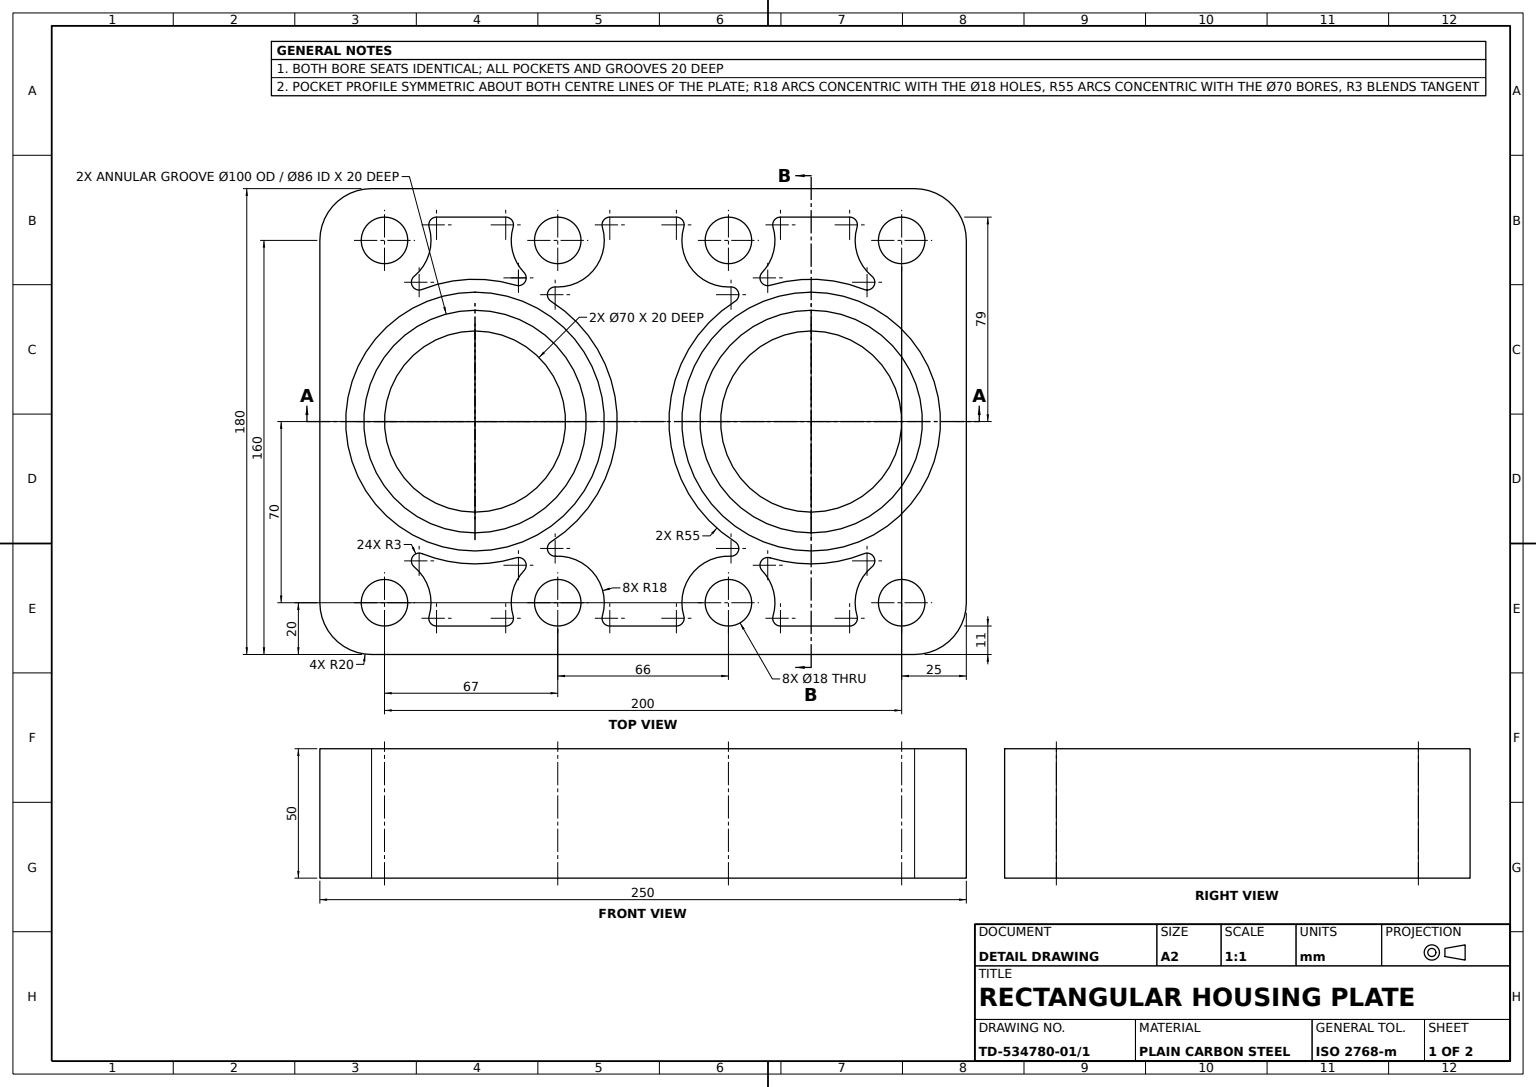
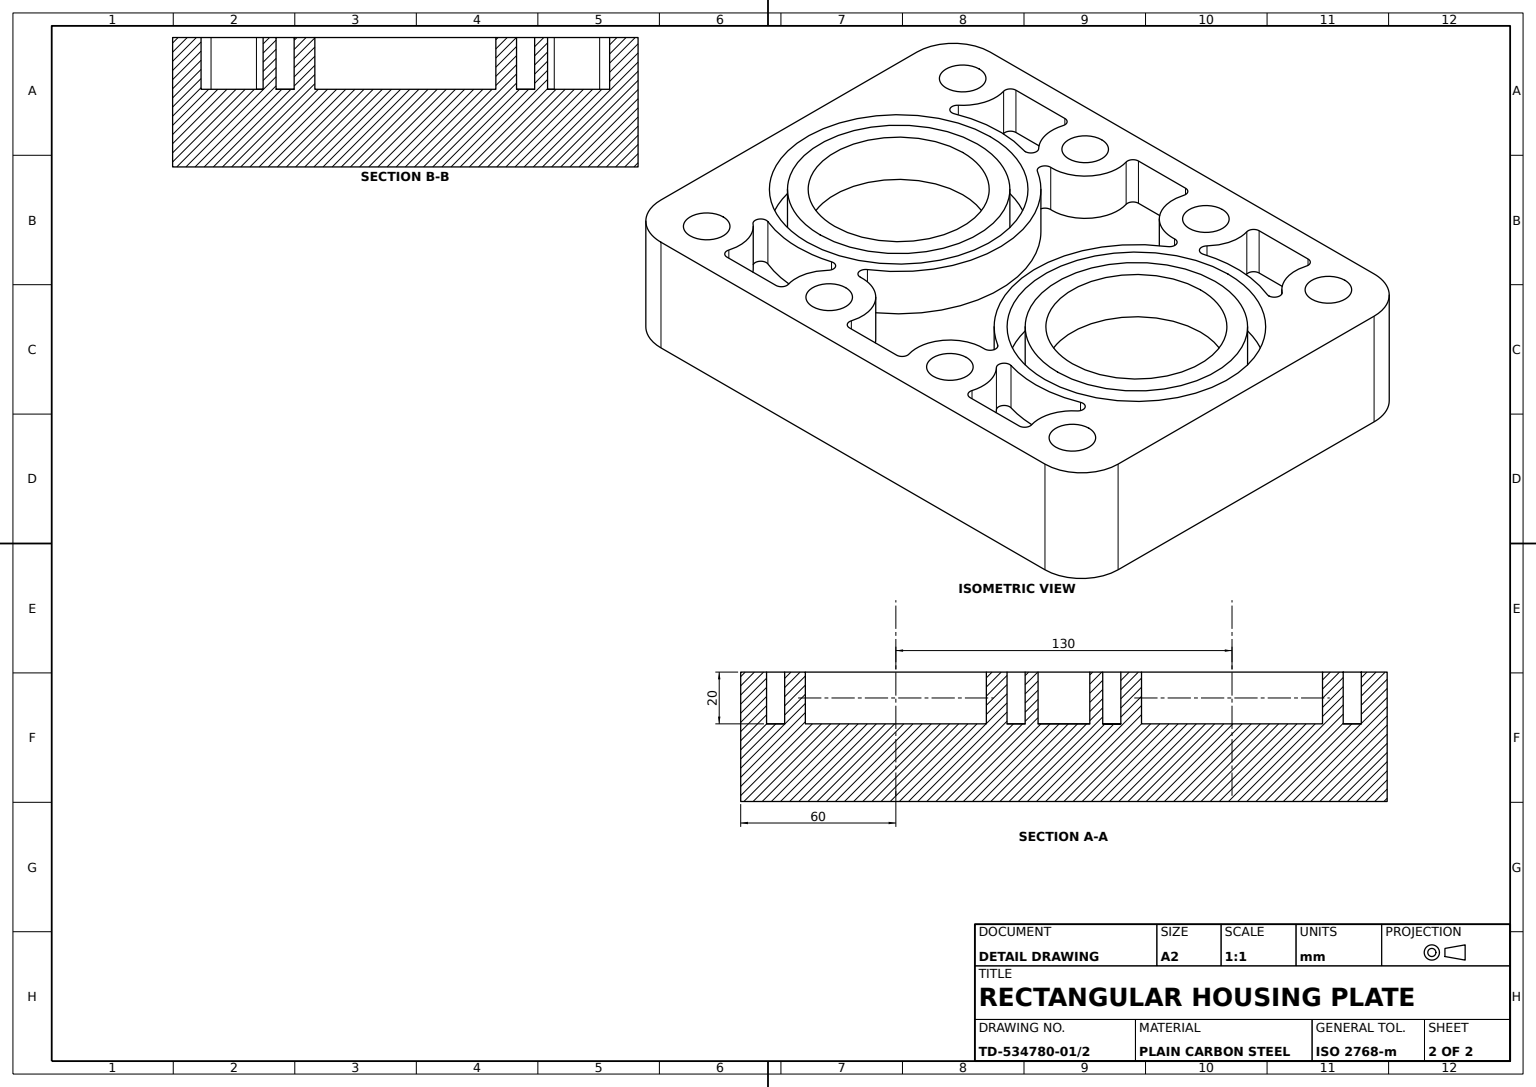
solid
v1 (100,0,61)
v2 (100,50,61)
e1 v1 v2 LINE
v3 (100,50,79)
e2 v2 v3 CIRCLE(AX(P(100,50,70),D(0,1,0),D(0,0,1)),9)
v4 (100,0,79)
e3 v4 v3 LINE
e4 v1 v4 CIRCLE(AX(P(100,0,70),D(0,1,0),D(0,0,1)),9)
face CYL(AX(P(100,-150,70),D(0,1,0),D(0,0,1)),9) rev [e1 e2 -e3 -e4]
v5 (65,30,-35)
v6 (65,30,35)
e5 v5 v6 CIRCLE(AX(P(65,30,0),D(0,1,0),D(0,0,1)),35)
e6 v6 v5 CIRCLE(AX(P(65,30,0),D(0,1,0),D(0,0,1)),35)
face PLANE(AX(P(0,30,0),D(0,1,0),D(0,0,1))) [e5 e6]
v7 (48.204819,30,-52.51506)
v8 (48.204819,50,-52.51506)
e7 v7 v8 LINE
v9 (49.073535,50,-52.643591)
e8 v8 v9 CIRCLE(AX(P(48.204819,50,-55.51506),D(0,1,0),D(0,0,1)),3)
v10 (49.073535,30,-52.643591)
e9 v10 v9 LINE
e10 v7 v10 CIRCLE(AX(P(48.204819,30,-55.51506),D(0,1,0),D(0,0,1)),3)
face CYL(AX(P(48.204819,30,-55.51506),D(0,1,0),D(0,0,1)),3) rev [e7 e8 -e9 -e10]
v11 (-125,50,-70)
v12 (-125,0,-70)
e11 v11 v12 LINE
v13 (-125,0,70)
e12 v12 v13 LINE
v14 (-125,50,70)
e13 v13 v14 LINE
e14 v11 v14 LINE
face PLANE(AX(P(-125,50,-90),D(1,0,0),D(0,0,-1))) rev [e11 e12 e13 -e14]
v15 (-33,0,61)
v16 (-33,50,61)
e15 v15 v16 LINE
v17 (-33,50,79)
e16 v16 v17 CIRCLE(AX(P(-33,50,70),D(0,1,0),D(0,0,1)),9)
v18 (-33,0,79)
e17 v18 v17 LINE
e18 v15 v18 CIRCLE(AX(P(-33,0,70),D(0,1,0),D(0,0,1)),9)
face CYL(AX(P(-33,-150,70),D(0,1,0),D(0,0,1)),9) rev [e15 e16 -e17 -e18]
v19 (-65,50,-35)
v20 (-65,50,35)
e19 v19 v20 CIRCLE(AX(P(-65,50,0),D(0,1,0),D(0,0,1)),35)
v21 (-65,30,35)
e20 v21 v20 LINE
v22 (-65,30,-35)
e21 v22 v21 CIRCLE(AX(P(-65,30,0),D(0,1,0),D(0,0,1)),35)
e22 v22 v19 LINE
face CYL(AX(P(-65,30,0),D(0,1,0),D(0,0,1)),35) rev [e19 -e20 -e21 e22]
v23 (-100,0,-61)
v24 (-100,50,-61)
e23 v23 v24 LINE
v25 (-100,50,-79)
e24 v24 v25 CIRCLE(AX(P(-100,50,-70),D(0,1,0),D(0,0,1)),9)
v26 (-100,0,-79)
e25 v26 v25 LINE
e26 v23 v26 CIRCLE(AX(P(-100,0,-70),D(0,1,0),D(0,0,1)),9)
face CYL(AX(P(-100,-150,-70),D(0,1,0),D(0,0,1)),9) rev [e23 e24 -e25 -e26]
v27 (-46.032702,30,57.584337)
v28 (-46.032702,50,57.584337)
e27 v27 v28 LINE
v29 (-49.073535,50,52.643591)
e28 v29 v28 CIRCLE(AX(P(-48.204819,50,55.51506),D(0,-1,0),D(0,0,1)),3)
v30 (-49.073535,30,52.643591)
e29 v30 v29 LINE
e30 v30 v27 CIRCLE(AX(P(-48.204819,30,55.51506),D(0,-1,0),D(0,0,1)),3)
face CYL(AX(P(-48.204819,30,55.51506),D(0,1,0),D(0,0,1)),3) rev [e27 -e28 -e29 e30]
v31 (-79.875388,30,79)
v32 (-79.875388,50,79)
e31 v31 v32 LINE
v33 (-82.750333,30,75.142857)
e32 v31 v33 CIRCLE(AX(P(-79.875388,30,76),D(0,-1,0),D(0,0,1)),3)
v34 (-82.750333,50,75.142857)
e33 v33 v34 LINE
e34 v32 v34 CIRCLE(AX(P(-79.875388,50,76),D(0,-1,0),D(0,0,1)),3)
face CYL(AX(P(-79.875388,30,76),D(0,1,0),D(0,0,1)),3) rev [-e31 e32 e33 -e34]
v35 (65,30,43)
v36 (65,30,-43)
e35 v35 v36 CIRCLE(AX(P(65,30,0),D(0,1,0),D(0,0,1)),43)
e36 v36 v35 CIRCLE(AX(P(65,30,0),D(0,1,0),D(0,0,1)),43)
v37 (65,30,50)
v38 (65,30,-50)
e37 v37 v38 CIRCLE(AX(P(65,30,0),D(0,1,0),D(0,0,1)),50)
e38 v38 v37 CIRCLE(AX(P(65,30,0),D(0,1,0),D(0,0,1)),50)
face PLANE(AX(P(0,30,0),D(0,1,0),D(0,0,1))) [-e35 -e36] [e37 e38]
v39 (35.608995,30,-46.488373)
v40 (35.608995,30,46.488373)
e39 v39 v40 CIRCLE(AX(P(65,30,0),D(0,1,0),D(0,0,1)),55)
v41 (35.608995,50,46.488373)
e40 v40 v41 LINE
v42 (35.608995,50,-46.488373)
e41 v42 v41 CIRCLE(AX(P(65,50,0),D(0,1,0),D(0,0,1)),55)
e42 v39 v42 LINE
face CYL(AX(P(65,30,0),D(0,1,0),D(0,0,1)),55) [e39 e40 -e41 -e42]
v43 (-48.204819,30,-52.51506)
v44 (-48.204819,50,-52.51506)
e43 v43 v44 LINE
v45 (-49.073535,30,-52.643591)
e44 v45 v43 CIRCLE(AX(P(-48.204819,30,-55.51506),D(0,1,0),D(0,0,1)),3)
v46 (-49.073535,50,-52.643591)
e45 v45 v46 LINE
e46 v46 v44 CIRCLE(AX(P(-48.204819,50,-55.51506),D(0,1,0),D(0,0,1)),3)
face CYL(AX(P(-48.204819,30,-55.51506),D(0,1,0),D(0,0,1)),3) rev [-e43 -e44 e45 e46]
v47 (33,0,-79)
v48 (33,50,-79)
e47 v47 v48 LINE
v49 (33,0,-61)
e48 v49 v47 CIRCLE(AX(P(33,0,-70),D(0,1,0),D(0,0,1)),9)
v50 (33,50,-61)
e49 v49 v50 LINE
e50 v50 v48 CIRCLE(AX(P(33,50,-70),D(0,1,0),D(0,0,1)),9)
face CYL(AX(P(33,-150,-70),D(0,1,0),D(0,0,1)),9) rev [-e47 -e48 e49 e50]
v51 (-50.249667,30,75.142857)
v52 (-53.124612,30,79)
e51 v51 v52 CIRCLE(AX(P(-53.124612,30,76),D(0,-1,0),D(0,0,1)),3)
e52 v27 v51 CIRCLE(AX(P(-33,30,70),D(0,1,0),D(0,0,1)),18)
v53 (-65,30,55)
e53 v53 v30 CIRCLE(AX(P(-65,30,0),D(0,1,0),D(0,0,1)),55)
v54 (-85.489465,30,51.040982)
e54 v54 v53 CIRCLE(AX(P(-65,30,0),D(0,1,0),D(0,0,1)),55)
v55 (-88.520347,30,56.135745)
e55 v55 v54 CIRCLE(AX(P(-86.607072,30,53.825035),D(0,-1,0),D(0,0,1)),3)
e56 v33 v55 CIRCLE(AX(P(-100,30,70),D(0,1,0),D(0,0,1)),18)
e57 v52 v31 LINE
face PLANE(AX(P(0,30,0),D(0,1,0),D(0,0,1))) [-e51 -e52 -e30 -e53 -e54 -e55 -e56 -e32 -e57]
v56 (65,30,55)
v57 (85.489465,30,51.040982)
e58 v56 v57 CIRCLE(AX(P(65,30,0),D(0,1,0),D(0,0,1)),55)
v58 (85.489465,50,51.040982)
e59 v57 v58 LINE
v59 (65,50,55)
e60 v59 v58 CIRCLE(AX(P(65,50,0),D(0,1,0),D(0,0,1)),55)
e61 v56 v59 LINE
face CYL(AX(P(65,30,0),D(0,1,0),D(0,0,1)),55) [e58 e59 -e60 -e61]
v60 (88.520347,30,56.135745)
e62 v57 v60 CIRCLE(AX(P(86.607072,30,53.825035),D(0,-1,0),D(0,0,1)),3)
v61 (88.520347,50,56.135745)
e63 v60 v61 LINE
e64 v58 v61 CIRCLE(AX(P(86.607072,50,53.825035),D(0,-1,0),D(0,0,1)),3)
face CYL(AX(P(86.607072,30,53.825035),D(0,1,0),D(0,0,1)),3) rev [-e59 e62 e63 -e64]
v62 (-35.608995,30,-46.488373)
v63 (-35.608995,50,-46.488373)
e65 v62 v63 LINE
v64 (-35.608995,50,46.488373)
e66 v64 v63 CIRCLE(AX(P(-65,50,0),D(0,1,0),D(0,0,1)),55)
v65 (-35.608995,30,46.488373)
e67 v65 v64 LINE
e68 v65 v62 CIRCLE(AX(P(-65,30,0),D(0,1,0),D(0,0,1)),55)
face CYL(AX(P(-65,30,0),D(0,1,0),D(0,0,1)),55) [e65 -e66 -e67 e68]
v66 (65,50,43)
e69 v35 v66 LINE
v67 (65,50,-43)
e70 v67 v66 CIRCLE(AX(P(65,50,0),D(0,1,0),D(0,0,1)),43)
e71 v36 v67 LINE
face CYL(AX(P(65,30,0),D(0,1,0),D(0,0,1)),43) [e36 e69 -e70 -e71]
v68 (15.750333,30,-75.142857)
v69 (12.875388,30,-79)
e72 v68 v69 CIRCLE(AX(P(12.875388,30,-76),D(0,1,0),D(0,0,1)),3)
v70 (15.750333,50,-75.142857)
e73 v68 v70 LINE
v71 (12.875388,50,-79)
e74 v70 v71 CIRCLE(AX(P(12.875388,50,-76),D(0,1,0),D(0,0,1)),3)
e75 v69 v71 LINE
face CYL(AX(P(12.875388,30,-76),D(0,1,0),D(0,0,1)),3) rev [-e72 e73 e74 -e75]
v72 (33,0,79)
v73 (33,50,79)
e76 v72 v73 LINE
v74 (33,50,61)
e77 v73 v74 CIRCLE(AX(P(33,50,70),D(0,1,0),D(0,0,1)),9)
v75 (33,0,61)
e78 v75 v74 LINE
e79 v72 v75 CIRCLE(AX(P(33,0,70),D(0,1,0),D(0,0,1)),9)
face CYL(AX(P(33,-150,70),D(0,1,0),D(0,0,1)),9) rev [e76 e77 -e78 -e79]
v76 (53.124612,30,-79)
v77 (50.249667,30,-75.142857)
e80 v76 v77 CIRCLE(AX(P(53.124612,30,-76),D(0,1,0),D(0,0,1)),3)
v78 (46.032702,30,-57.584337)
e81 v78 v77 CIRCLE(AX(P(33,30,-70),D(0,1,0),D(0,0,1)),18)
e82 v78 v7 CIRCLE(AX(P(48.204819,30,-55.51506),D(0,1,0),D(0,0,1)),3)
v79 (85.489465,30,-51.040982)
e83 v79 v10 CIRCLE(AX(P(65,30,0),D(0,1,0),D(0,0,1)),55)
v80 (86.607072,30,-50.825035)
e84 v79 v80 CIRCLE(AX(P(86.607072,30,-53.825035),D(0,1,0),D(0,0,1)),3)
v81 (88.520347,30,-56.135745)
e85 v80 v81 CIRCLE(AX(P(86.607072,30,-53.825035),D(0,1,0),D(0,0,1)),3)
v82 (82.750333,30,-75.142857)
e86 v82 v81 CIRCLE(AX(P(100,30,-70),D(0,1,0),D(0,0,1)),18)
v83 (79.875388,30,-79)
e87 v82 v83 CIRCLE(AX(P(79.875388,30,-76),D(0,1,0),D(0,0,1)),3)
e88 v76 v83 LINE
face PLANE(AX(P(0,30,0),D(0,1,0),D(0,0,1))) [e80 -e81 e82 e10 -e83 e84 e85 -e86 e87 -e88]
v84 (65,50,50)
v85 (65,50,-50)
e89 v84 v85 CIRCLE(AX(P(65,50,0),D(0,1,0),D(0,0,1)),50)
e90 v38 v85 LINE
e91 v37 v84 LINE
face CYL(AX(P(65,30,0),D(0,1,0),D(0,0,1)),50) rev [e89 -e90 -e37 e91]
v86 (-65,30,-50)
v87 (-65,30,50)
e92 v86 v87 CIRCLE(AX(P(-65,30,0),D(0,1,0),D(0,0,1)),50)
e93 v87 v86 CIRCLE(AX(P(-65,30,0),D(0,1,0),D(0,0,1)),50)
v88 (-65,30,-43)
v89 (-65,30,43)
e94 v88 v89 CIRCLE(AX(P(-65,30,0),D(0,1,0),D(0,0,1)),43)
e95 v89 v88 CIRCLE(AX(P(-65,30,0),D(0,1,0),D(0,0,1)),43)
face PLANE(AX(P(0,30,0),D(0,1,0),D(0,0,1))) [e92 e93] [-e94 -e95]
v90 (-33,50,-52)
v91 (-33.862157,50,-52.020659)
e96 v90 v91 CIRCLE(AX(P(-33,50,-70),D(0,-1,0),D(0,0,1)),18)
v92 (-33.862157,30,-52.020659)
e97 v92 v91 LINE
v93 (-33,30,-52)
e98 v93 v92 CIRCLE(AX(P(-33,30,-70),D(0,-1,0),D(0,0,1)),18)
e99 v93 v90 LINE
face CYL(AX(P(-33,30,-70),D(0,1,0),D(0,0,1)),18) [e96 -e97 -e98 e99]
v94 (-53.124612,50,79)
e100 v94 v32 LINE
e101 v52 v94 LINE
face PLANE(AX(P(0,30,79),D(0,0,-1),D(-1,0,0))) [e57 e31 -e100 -e101]
v95 (65,50,-35)
e102 v5 v95 LINE
v96 (65,50,35)
e103 v6 v96 LINE
e104 v96 v95 CIRCLE(AX(P(65,50,0),D(0,1,0),D(0,0,1)),35)
face CYL(AX(P(65,30,0),D(0,1,0),D(0,0,1)),35) rev [-e102 -e6 e103 e104]
v97 (-50.249667,50,75.142857)
e105 v97 v94 CIRCLE(AX(P(-53.124612,50,76),D(0,-1,0),D(0,0,1)),3)
e106 v51 v97 LINE
face CYL(AX(P(-53.124612,30,76),D(0,1,0),D(0,0,1)),3) rev [-e105 -e106 e51 e101]
v98 (88.520347,50,-56.135745)
e107 v81 v98 LINE
v99 (86.607072,50,-50.825035)
e108 v80 v99 LINE
e109 v99 v98 CIRCLE(AX(P(86.607072,50,-53.825035),D(0,1,0),D(0,0,1)),3)
face CYL(AX(P(86.607072,30,-53.825035),D(0,1,0),D(0,0,1)),3) rev [-e107 -e85 e108 e109]
e110 v21 v22 CIRCLE(AX(P(-65,30,0),D(0,1,0),D(0,0,1)),35)
e111 v20 v19 CIRCLE(AX(P(-65,50,0),D(0,1,0),D(0,0,1)),35)
face CYL(AX(P(-65,30,0),D(0,1,0),D(0,0,1)),35) rev [-e110 e20 e111 -e22]
e112 v47 v49 CIRCLE(AX(P(33,0,-70),D(0,1,0),D(0,0,1)),9)
e113 v48 v50 CIRCLE(AX(P(33,50,-70),D(0,1,0),D(0,0,1)),9)
face CYL(AX(P(33,-150,-70),D(0,1,0),D(0,0,1)),9) rev [-e49 -e112 e47 e113]
v100 (-12.875388,50,-79)
e114 v100 v71 LINE
v101 (-12.875388,30,-79)
e115 v101 v100 LINE
e116 v101 v69 LINE
face PLANE(AX(P(0,30,-79),D(0,0,1),D(1,0,0))) [e75 -e114 -e115 e116]
v102 (33.862157,50,-52.020659)
e117 v42 v102 CIRCLE(AX(P(34.00585,50,-49.024103),D(0,1,0),D(0,0,1)),3)
v103 (33.862157,30,-52.020659)
e118 v103 v102 LINE
e119 v39 v103 CIRCLE(AX(P(34.00585,30,-49.024103),D(0,1,0),D(0,0,1)),3)
face CYL(AX(P(34.00585,30,-49.024103),D(0,1,0),D(0,0,1)),3) rev [e42 e117 -e118 -e119]
v104 (-65,50,55)
e120 v104 v29 CIRCLE(AX(P(-65,50,0),D(0,1,0),D(0,0,1)),55)
e121 v53 v104 LINE
face CYL(AX(P(-65,30,0),D(0,1,0),D(0,0,1)),55) [e29 -e120 -e121 e53]
v105 (-34.00585,30,52.024103)
e122 v105 v65 CIRCLE(AX(P(-34.00585,30,49.024103),D(0,-1,0),D(0,0,1)),3)
v106 (-34.00585,50,52.024103)
e123 v106 v64 CIRCLE(AX(P(-34.00585,50,49.024103),D(0,-1,0),D(0,0,1)),3)
e124 v105 v106 LINE
face CYL(AX(P(-34.00585,30,49.024103),D(0,1,0),D(0,0,1)),3) rev [e122 e67 -e123 -e124]
v107 (105,50,-90)
v108 (105,0,-90)
e125 v107 v108 LINE
v109 (-105,0,-90)
e126 v108 v109 LINE
v110 (-105,50,-90)
e127 v109 v110 LINE
e128 v107 v110 LINE
face PLANE(AX(P(125,50,-90),D(0,0,1),D(1,0,0))) rev [e125 e126 e127 -e128]
v111 (-100,0,79)
v112 (-100,50,79)
e129 v111 v112 LINE
v113 (-100,50,61)
e130 v112 v113 CIRCLE(AX(P(-100,50,70),D(0,1,0),D(0,0,1)),9)
v114 (-100,0,61)
e131 v114 v113 LINE
e132 v111 v114 CIRCLE(AX(P(-100,0,70),D(0,1,0),D(0,0,1)),9)
face CYL(AX(P(-100,-150,70),D(0,1,0),D(0,0,1)),9) rev [e129 e130 -e131 -e132]
v115 (-79.875388,30,-79)
v116 (-79.875388,50,-79)
e133 v115 v116 LINE
v117 (-53.124612,30,-79)
e134 v117 v115 LINE
v118 (-53.124612,50,-79)
e135 v117 v118 LINE
e136 v118 v116 LINE
face PLANE(AX(P(0,30,-79),D(0,0,-1),D(-1,0,0))) rev [-e133 -e134 e135 e136]
v119 (85.489465,50,-51.040982)
e137 v119 v9 CIRCLE(AX(P(65,50,0),D(0,1,0),D(0,0,1)),55)
e138 v79 v119 LINE
face CYL(AX(P(65,30,0),D(0,1,0),D(0,0,1)),55) [e83 e9 -e137 -e138]
e139 v66 v67 CIRCLE(AX(P(65,50,0),D(0,1,0),D(0,0,1)),43)
e140 v95 v96 CIRCLE(AX(P(65,50,0),D(0,1,0),D(0,0,1)),35)
face PLANE(AX(P(0,50,0),D(0,1,0),D(0,0,1))) [e70 e139] [-e104 -e140]
v120 (53.124612,30,79)
v121 (53.124612,50,79)
e141 v120 v121 LINE
v122 (50.249667,30,75.142857)
e142 v120 v122 CIRCLE(AX(P(53.124612,30,76),D(0,-1,0),D(0,0,1)),3)
v123 (50.249667,50,75.142857)
e143 v122 v123 LINE
e144 v121 v123 CIRCLE(AX(P(53.124612,50,76),D(0,-1,0),D(0,0,1)),3)
face CYL(AX(P(53.124612,30,76),D(0,1,0),D(0,0,1)),3) rev [-e141 e142 e143 -e144]
v124 (-50.249667,30,-75.142857)
e145 v124 v117 CIRCLE(AX(P(-53.124612,30,-76),D(0,1,0),D(0,0,1)),3)
v125 (-50.249667,50,-75.142857)
e146 v124 v125 LINE
e147 v125 v118 CIRCLE(AX(P(-53.124612,50,-76),D(0,1,0),D(0,0,1)),3)
face CYL(AX(P(-53.124612,30,-76),D(0,1,0),D(0,0,1)),3) rev [-e145 e146 e147 -e135]
v126 (49.073535,30,52.643591)
e148 v126 v56 CIRCLE(AX(P(65,30,0),D(0,1,0),D(0,0,1)),55)
v127 (46.032702,30,57.584337)
e149 v127 v126 CIRCLE(AX(P(48.204819,30,55.51506),D(0,-1,0),D(0,0,1)),3)
e150 v127 v122 CIRCLE(AX(P(33,30,70),D(0,-1,0),D(0,0,1)),18)
v128 (79.875388,30,79)
e151 v120 v128 LINE
v129 (82.750333,30,75.142857)
e152 v129 v128 CIRCLE(AX(P(79.875388,30,76),D(0,-1,0),D(0,0,1)),3)
e153 v129 v60 CIRCLE(AX(P(100,30,70),D(0,-1,0),D(0,0,1)),18)
face PLANE(AX(P(0,30,0),D(0,1,0),D(0,0,1))) [-e62 -e58 -e148 -e149 e150 -e142 e151 -e152 e153]
v130 (53.124612,50,-79)
e154 v76 v130 LINE
v131 (50.249667,50,-75.142857)
e155 v130 v131 CIRCLE(AX(P(53.124612,50,-76),D(0,1,0),D(0,0,1)),3)
e156 v77 v131 LINE
face CYL(AX(P(53.124612,30,-76),D(0,1,0),D(0,0,1)),3) rev [-e80 e154 e155 -e156]
v132 (-85.489465,50,51.040982)
e157 v54 v132 LINE
v133 (-88.520347,50,56.135745)
e158 v133 v132 CIRCLE(AX(P(-86.607072,50,53.825035),D(0,-1,0),D(0,0,1)),3)
e159 v55 v133 LINE
face CYL(AX(P(-86.607072,30,53.825035),D(0,1,0),D(0,0,1)),3) rev [e157 -e158 -e159 e55]
v134 (82.750333,50,-75.142857)
e160 v134 v98 CIRCLE(AX(P(100,50,-70),D(0,1,0),D(0,0,1)),18)
e161 v82 v134 LINE
face CYL(AX(P(100,30,-70),D(0,1,0),D(0,0,1)),18) [e86 e107 -e160 -e161]
v135 (79.875388,50,79)
e162 v128 v135 LINE
v136 (82.750333,50,75.142857)
e163 v136 v135 CIRCLE(AX(P(79.875388,50,76),D(0,-1,0),D(0,0,1)),3)
e164 v129 v136 LINE
face CYL(AX(P(79.875388,30,76),D(0,1,0),D(0,0,1)),3) rev [e152 e162 -e163 -e164]
v137 (100,50,-79)
v138 (100,50,-61)
e165 v137 v138 CIRCLE(AX(P(100,50,-70),D(0,1,0),D(0,0,1)),9)
v139 (100,0,-61)
e166 v139 v138 LINE
v140 (100,0,-79)
e167 v140 v139 CIRCLE(AX(P(100,0,-70),D(0,1,0),D(0,0,1)),9)
e168 v140 v137 LINE
face CYL(AX(P(100,-150,-70),D(0,1,0),D(0,0,1)),9) rev [e165 -e166 -e167 e168]
v141 (-65,50,50)
e169 v87 v141 LINE
v142 (-65,50,-50)
e170 v141 v142 CIRCLE(AX(P(-65,50,0),D(0,1,0),D(0,0,1)),50)
e171 v86 v142 LINE
face CYL(AX(P(-65,30,0),D(0,1,0),D(0,0,1)),50) rev [e169 e170 -e171 -e93]
v143 (46.032702,50,-57.584337)
e172 v143 v131 CIRCLE(AX(P(33,50,-70),D(0,1,0),D(0,0,1)),18)
e173 v78 v143 LINE
face CYL(AX(P(33,30,-70),D(0,1,0),D(0,0,1)),18) [e156 -e172 -e173 e81]
v144 (125,50,-70)
e174 v144 v107 CIRCLE(AX(P(105,50,-70),D(0,1,0),D(0,0,1)),20)
v145 (125,0,-70)
e175 v145 v144 LINE
e176 v108 v145 CIRCLE(AX(P(105,0,-70),D(0,-1,0),D(0,0,1)),20)
face CYL(AX(P(105,50,-70),D(0,-1,0),D(0,0,-1)),20) [-e125 -e174 -e175 -e176]
e177 v91 v63 CIRCLE(AX(P(-34.00585,50,-49.024103),D(0,1,0),D(0,0,1)),3)
e178 v92 v62 CIRCLE(AX(P(-34.00585,30,-49.024103),D(0,1,0),D(0,0,1)),3)
face CYL(AX(P(-34.00585,30,-49.024103),D(0,1,0),D(0,0,1)),3) rev [e97 e177 -e65 -e178]
e179 v114 v111 CIRCLE(AX(P(-100,0,70),D(0,1,0),D(0,0,1)),9)
e180 v113 v112 CIRCLE(AX(P(-100,50,70),D(0,1,0),D(0,0,1)),9)
face CYL(AX(P(-100,-150,70),D(0,1,0),D(0,0,1)),9) rev [-e179 e131 e180 -e129]
v146 (79.875388,50,-79)
e181 v134 v146 CIRCLE(AX(P(79.875388,50,-76),D(0,1,0),D(0,0,1)),3)
e182 v83 v146 LINE
face CYL(AX(P(79.875388,30,-76),D(0,1,0),D(0,0,1)),3) rev [e161 e181 -e182 -e87]
v147 (-105,0,90)
e183 v147 v13 CIRCLE(AX(P(-105,0,70),D(0,-1,0),D(0,0,1)),20)
v148 (-105,50,90)
e184 v148 v147 LINE
e185 v14 v148 CIRCLE(AX(P(-105,50,70),D(0,1,0),D(0,0,1)),20)
face CYL(AX(P(-105,50,70),D(0,-1,0),D(0,0,-1)),20) [-e183 -e184 -e185 -e13]
e186 v18 v15 CIRCLE(AX(P(-33,0,70),D(0,1,0),D(0,0,1)),9)
e187 v139 v140 CIRCLE(AX(P(100,0,-70),D(0,1,0),D(0,0,1)),9)
e188 v75 v72 CIRCLE(AX(P(33,0,70),D(0,1,0),D(0,0,1)),9)
e189 v4 v1 CIRCLE(AX(P(100,0,70),D(0,1,0),D(0,0,1)),9)
v149 (105,0,90)
e190 v147 v149 LINE
e191 v12 v109 CIRCLE(AX(P(-105,0,-70),D(0,-1,0),D(0,0,1)),20)
v150 (125,0,70)
e192 v150 v145 LINE
e193 v150 v149 CIRCLE(AX(P(105,0,70),D(0,-1,0),D(0,0,1)),20)
e194 v26 v23 CIRCLE(AX(P(-100,0,-70),D(0,1,0),D(0,0,1)),9)
v151 (-33,0,-61)
v152 (-33,0,-79)
e195 v151 v152 CIRCLE(AX(P(-33,0,-70),D(0,1,0),D(0,0,1)),9)
e196 v152 v151 CIRCLE(AX(P(-33,0,-70),D(0,1,0),D(0,0,1)),9)
face PLANE(AX(P(0,0,0),D(0,1,0),D(0,0,1))) rev [e186 e18] [e179 e132] [e187 e167] [e188 e79] [e189 e4] [-e190 e183 -e12 e191 -e126 e176 -e192 e193] [e194 e26] [e195 e196] [e112 e48]
v153 (125,50,70)
e197 v153 v144 LINE
e198 v153 v150 LINE
face PLANE(AX(P(125,50,0),D(-1,0,0),D(0,0,1))) rev [e175 -e197 e198 e192]
v154 (-82.750333,30,-75.142857)
v155 (-88.520347,30,-56.135745)
e199 v154 v155 CIRCLE(AX(P(-100,30,-70),D(0,-1,0),D(0,0,1)),18)
v156 (-86.607072,30,-50.825035)
e200 v155 v156 CIRCLE(AX(P(-86.607072,30,-53.825035),D(0,1,0),D(0,0,1)),3)
v157 (-85.489465,30,-51.040982)
e201 v156 v157 CIRCLE(AX(P(-86.607072,30,-53.825035),D(0,1,0),D(0,0,1)),3)
e202 v45 v157 CIRCLE(AX(P(-65,30,0),D(0,1,0),D(0,0,1)),55)
v158 (-46.032702,30,-57.584337)
e203 v43 v158 CIRCLE(AX(P(-48.204819,30,-55.51506),D(0,1,0),D(0,0,1)),3)
e204 v158 v124 CIRCLE(AX(P(-33,30,-70),D(0,-1,0),D(0,0,1)),18)
e205 v115 v154 CIRCLE(AX(P(-79.875388,30,-76),D(0,1,0),D(0,0,1)),3)
face PLANE(AX(P(0,30,0),D(0,1,0),D(0,0,1))) [e199 e200 e201 -e202 e44 e203 e204 e145 e134 e205]
v159 (12.875388,30,79)
v160 (12.875388,50,79)
e206 v159 v160 LINE
v161 (15.750333,50,75.142857)
e207 v161 v160 CIRCLE(AX(P(12.875388,50,76),D(0,-1,0),D(0,0,1)),3)
v162 (15.750333,30,75.142857)
e208 v162 v161 LINE
e209 v162 v159 CIRCLE(AX(P(12.875388,30,76),D(0,-1,0),D(0,0,1)),3)
face CYL(AX(P(12.875388,30,76),D(0,1,0),D(0,0,1)),3) rev [e206 -e207 -e208 e209]
v163 (46.032702,50,57.584337)
e210 v127 v163 LINE
e211 v163 v123 CIRCLE(AX(P(33,50,70),D(0,-1,0),D(0,0,1)),18)
face CYL(AX(P(33,30,70),D(0,1,0),D(0,0,1)),18) [e210 e211 -e143 -e150]
v164 (-33,50,-61)
e212 v151 v164 LINE
v165 (-33,50,-79)
e213 v164 v165 CIRCLE(AX(P(-33,50,-70),D(0,1,0),D(0,0,1)),9)
e214 v152 v165 LINE
face CYL(AX(P(-33,-150,-70),D(0,1,0),D(0,0,1)),9) rev [-e195 e212 e213 -e214]
v166 (-15.750333,50,-75.142857)
e215 v100 v166 CIRCLE(AX(P(-12.875388,50,-76),D(0,1,0),D(0,0,1)),3)
v167 (-15.750333,30,-75.142857)
e216 v167 v166 LINE
e217 v101 v167 CIRCLE(AX(P(-12.875388,30,-76),D(0,1,0),D(0,0,1)),3)
face CYL(AX(P(-12.875388,30,-76),D(0,1,0),D(0,0,1)),3) rev [e115 e215 -e216 -e217]
e218 v3 v2 CIRCLE(AX(P(100,50,70),D(0,1,0),D(0,0,1)),9)
face CYL(AX(P(100,-150,70),D(0,1,0),D(0,0,1)),9) rev [-e1 -e189 e3 e218]
e219 v34 v133 CIRCLE(AX(P(-100,50,70),D(0,1,0),D(0,0,1)),18)
face CYL(AX(P(-100,30,70),D(0,1,0),D(0,0,1)),18) [-e33 e56 e159 -e219]
v168 (-46.032702,50,-57.584337)
e220 v44 v168 CIRCLE(AX(P(-48.204819,50,-55.51506),D(0,1,0),D(0,0,1)),3)
e221 v158 v168 LINE
face CYL(AX(P(-48.204819,30,-55.51506),D(0,1,0),D(0,0,1)),3) rev [e220 -e221 -e203 e43]
v169 (-88.520347,50,-56.135745)
e222 v155 v169 LINE
v170 (-82.750333,50,-75.142857)
e223 v154 v170 LINE
e224 v170 v169 CIRCLE(AX(P(-100,50,-70),D(0,-1,0),D(0,0,1)),18)
face CYL(AX(P(-100,30,-70),D(0,1,0),D(0,0,1)),18) [-e222 -e199 e223 e224]
e225 v25 v24 CIRCLE(AX(P(-100,50,-70),D(0,1,0),D(0,0,1)),9)
face CYL(AX(P(-100,-150,-70),D(0,1,0),D(0,0,1)),9) rev [-e194 e25 e225 -e23]
face CYL(AX(P(65,30,0),D(0,1,0),D(0,0,1)),35) rev [-e103 -e5 e102 e140]
e226 v17 v16 CIRCLE(AX(P(-33,50,70),D(0,1,0),D(0,0,1)),9)
face CYL(AX(P(-33,-150,70),D(0,1,0),D(0,0,1)),9) rev [e226 -e15 -e186 e17]
v171 (33,30,-52)
e227 v68 v171 CIRCLE(AX(P(33,30,-70),D(0,1,0),D(0,0,1)),18)
v172 (33,50,-52)
e228 v171 v172 LINE
e229 v70 v172 CIRCLE(AX(P(33,50,-70),D(0,1,0),D(0,0,1)),18)
face CYL(AX(P(33,30,-70),D(0,1,0),D(0,0,1)),18) [-e73 e227 e228 -e229]
v173 (-65,50,-43)
v174 (-65,50,43)
e230 v173 v174 CIRCLE(AX(P(-65,50,0),D(0,1,0),D(0,0,1)),43)
e231 v174 v173 CIRCLE(AX(P(-65,50,0),D(0,1,0),D(0,0,1)),43)
face PLANE(AX(P(0,50,0),D(0,1,0),D(0,0,1))) [-e19 -e111] [e230 e231]
e232 v136 v61 CIRCLE(AX(P(100,50,70),D(0,-1,0),D(0,0,1)),18)
face CYL(AX(P(100,30,70),D(0,1,0),D(0,0,1)),18) [-e153 e164 e232 -e63]
e233 v116 v170 CIRCLE(AX(P(-79.875388,50,-76),D(0,1,0),D(0,0,1)),3)
face CYL(AX(P(-79.875388,30,-76),D(0,1,0),D(0,0,1)),3) rev [-e205 e133 e233 -e223]
e234 v165 v164 CIRCLE(AX(P(-33,50,-70),D(0,1,0),D(0,0,1)),9)
face CYL(AX(P(-33,-150,-70),D(0,1,0),D(0,0,1)),9) rev [-e196 e214 e234 -e212]
face PLANE(AX(P(0,30,0),D(0,1,0),D(0,0,1))) [e110 e21]
face CYL(AX(P(65,30,0),D(0,1,0),D(0,0,1)),43) [-e69 e35 e71 -e139]
v175 (-86.607072,50,-50.825035)
e235 v169 v175 CIRCLE(AX(P(-86.607072,50,-53.825035),D(0,1,0),D(0,0,1)),3)
e236 v156 v175 LINE
face CYL(AX(P(-86.607072,30,-53.825035),D(0,1,0),D(0,0,1)),3) rev [-e200 e222 e235 -e236]
e237 v143 v8 CIRCLE(AX(P(48.204819,50,-55.51506),D(0,1,0),D(0,0,1)),3)
face CYL(AX(P(48.204819,30,-55.51506),D(0,1,0),D(0,0,1)),3) rev [e173 e237 -e7 -e82]
e238 v130 v146 LINE
face PLANE(AX(P(0,30,-79),D(0,0,1),D(1,0,0))) [e182 -e238 -e154 e88]
e239 v28 v97 CIRCLE(AX(P(-33,50,70),D(0,1,0),D(0,0,1)),18)
face CYL(AX(P(-33,30,70),D(0,1,0),D(0,0,1)),18) [-e239 -e27 e52 e106]
e240 v167 v93 CIRCLE(AX(P(-33,30,-70),D(0,-1,0),D(0,0,1)),18)
e241 v166 v90 CIRCLE(AX(P(-33,50,-70),D(0,-1,0),D(0,0,1)),18)
face CYL(AX(P(-33,30,-70),D(0,1,0),D(0,0,1)),18) [-e240 e216 e241 -e99]
e242 v171 v103 CIRCLE(AX(P(33,30,-70),D(0,1,0),D(0,0,1)),18)
v176 (-33.862157,30,52.020659)
e243 v176 v105 CIRCLE(AX(P(-34.00585,30,49.024103),D(0,-1,0),D(0,0,1)),3)
v177 (-15.750333,30,75.142857)
e244 v177 v176 CIRCLE(AX(P(-33,30,70),D(0,1,0),D(0,0,1)),18)
v178 (-12.875388,30,79)
e245 v178 v177 CIRCLE(AX(P(-12.875388,30,76),D(0,-1,0),D(0,0,1)),3)
e246 v159 v178 LINE
v179 (33.862157,30,52.020659)
e247 v162 v179 CIRCLE(AX(P(33,30,70),D(0,-1,0),D(0,0,1)),18)
v180 (34.00585,30,52.024103)
e248 v180 v179 CIRCLE(AX(P(34.00585,30,49.024103),D(0,-1,0),D(0,0,1)),3)
e249 v40 v180 CIRCLE(AX(P(34.00585,30,49.024103),D(0,-1,0),D(0,0,1)),3)
face PLANE(AX(P(0,30,0),D(0,1,0),D(0,0,1))) [-e39 e119 -e242 -e227 e72 -e116 e217 e240 e98 e178 -e68 -e122 -e243 -e244 -e245 -e246 -e209 e247 -e248 -e249]
e250 v168 v125 CIRCLE(AX(P(-33,50,-70),D(0,-1,0),D(0,0,1)),18)
face CYL(AX(P(-33,30,-70),D(0,1,0),D(0,0,1)),18) [-e204 e221 e250 -e146]
e251 v138 v137 CIRCLE(AX(P(100,50,-70),D(0,1,0),D(0,0,1)),9)
face CYL(AX(P(100,-150,-70),D(0,1,0),D(0,0,1)),9) rev [e166 e251 -e168 -e187]
e252 v121 v135 LINE
face PLANE(AX(P(0,30,79),D(0,0,1),D(1,0,0))) rev [-e151 e141 e252 -e162]
v181 (105,50,90)
e253 v181 v153 CIRCLE(AX(P(105,50,70),D(0,1,0),D(0,0,1)),20)
e254 v149 v181 LINE
face CYL(AX(P(105,50,70),D(0,-1,0),D(0,0,-1)),20) [-e198 -e253 -e254 -e193]
v182 (-85.489465,50,-51.040982)
e255 v157 v182 LINE
e256 v46 v182 CIRCLE(AX(P(-65,50,0),D(0,1,0),D(0,0,1)),55)
face CYL(AX(P(-65,30,0),D(0,1,0),D(0,0,1)),55) [e255 -e256 -e45 e202]
v183 (33.862157,50,52.020659)
e257 v161 v183 CIRCLE(AX(P(33,50,70),D(0,-1,0),D(0,0,1)),18)
e258 v179 v183 LINE
face CYL(AX(P(33,30,70),D(0,1,0),D(0,0,1)),18) [e208 e257 -e258 -e247]
e259 v85 v84 CIRCLE(AX(P(65,50,0),D(0,1,0),D(0,0,1)),50)
face CYL(AX(P(65,30,0),D(0,1,0),D(0,0,1)),50) rev [-e91 -e38 e90 e259]
e260 v89 v174 LINE
e261 v88 v173 LINE
face CYL(AX(P(-65,30,0),D(0,1,0),D(0,0,1)),43) [-e231 -e260 e95 e261]
e262 v142 v141 CIRCLE(AX(P(-65,50,0),D(0,1,0),D(0,0,1)),50)
face CYL(AX(P(-65,30,0),D(0,1,0),D(0,0,1)),50) rev [e262 -e169 -e92 e171]
v184 (-33.862157,50,52.020659)
e263 v176 v184 LINE
v185 (-15.750333,50,75.142857)
e264 v185 v184 CIRCLE(AX(P(-33,50,70),D(0,1,0),D(0,0,1)),18)
e265 v177 v185 LINE
face CYL(AX(P(-33,30,70),D(0,1,0),D(0,0,1)),18) [e263 -e264 -e265 e244]
e266 v132 v104 CIRCLE(AX(P(-65,50,0),D(0,1,0),D(0,0,1)),55)
face CYL(AX(P(-65,30,0),D(0,1,0),D(0,0,1)),55) [e121 -e266 -e157 e54]
e267 v175 v182 CIRCLE(AX(P(-86.607072,50,-53.825035),D(0,1,0),D(0,0,1)),3)
face CYL(AX(P(-86.607072,30,-53.825035),D(0,1,0),D(0,0,1)),3) rev [-e255 -e201 e236 e267]
v186 (-12.875388,50,79)
e268 v178 v186 LINE
e269 v160 v186 LINE
face PLANE(AX(P(0,30,79),D(0,0,-1),D(-1,0,0))) [e268 -e269 -e206 e246]
e270 v148 v181 LINE
face PLANE(AX(P(-125,50,90),D(0,0,-1),D(-1,0,0))) rev [e184 e190 e254 -e270]
e271 v119 v99 CIRCLE(AX(P(86.607072,50,-53.825035),D(0,1,0),D(0,0,1)),3)
face CYL(AX(P(86.607072,30,-53.825035),D(0,1,0),D(0,0,1)),3) rev [-e84 e138 e271 -e108]
e272 v110 v11 CIRCLE(AX(P(-105,50,-70),D(0,1,0),D(0,0,1)),20)
face CYL(AX(P(-105,50,-70),D(0,-1,0),D(0,0,-1)),20) [-e127 -e191 -e11 -e272]
v187 (49.073535,50,52.643591)
e273 v187 v59 CIRCLE(AX(P(65,50,0),D(0,1,0),D(0,0,1)),55)
e274 v126 v187 LINE
face CYL(AX(P(65,30,0),D(0,1,0),D(0,0,1)),55) [e148 e61 -e273 -e274]
v188 (34.00585,50,52.024103)
e275 v188 v183 CIRCLE(AX(P(34.00585,50,49.024103),D(0,-1,0),D(0,0,1)),3)
e276 v180 v188 LINE
face CYL(AX(P(34.00585,30,49.024103),D(0,1,0),D(0,0,1)),3) rev [e258 -e275 -e276 e248]
e277 v41 v188 CIRCLE(AX(P(34.00585,50,49.024103),D(0,-1,0),D(0,0,1)),3)
face CYL(AX(P(34.00585,30,49.024103),D(0,1,0),D(0,0,1)),3) rev [e249 e276 -e277 -e40]
e278 v184 v106 CIRCLE(AX(P(-34.00585,50,49.024103),D(0,-1,0),D(0,0,1)),3)
e279 v172 v102 CIRCLE(AX(P(33,50,-70),D(0,1,0),D(0,0,1)),18)
e280 v186 v185 CIRCLE(AX(P(-12.875388,50,76),D(0,-1,0),D(0,0,1)),3)
e281 v74 v73 CIRCLE(AX(P(33,50,70),D(0,1,0),D(0,0,1)),9)
e282 v163 v187 CIRCLE(AX(P(48.204819,50,55.51506),D(0,-1,0),D(0,0,1)),3)
face PLANE(AX(P(0,50,0),D(0,1,0),D(0,0,1))) [e278 e123 e66 -e177 -e96 -e241 -e215 e114 -e74 e229 e279 -e117 e41 e277 e275 -e257 e207 e269 e280 e264] [-e267 -e235 -e224 -e233 -e136 -e147 -e250 -e220 -e46 e256] [-e251 -e165] [-e77 -e281] [e185 e270 e253 e197 e174 e128 e272 e14] [-e218 -e2] [-e259 -e89] [e282 e273 e60 e64 -e232 e163 -e252 e144 -e211] [-e225 -e24] [e34 e219 e158 e266 e120 e28 e239 e105 e100] [-e180 -e130] [-e16 -e226] [-e50 -e113] [-e271 e137 -e8 -e237 e172 -e155 e238 -e181 e160 -e109] [-e213 -e234] [-e170 -e262]
face CYL(AX(P(48.204819,30,55.51506),D(0,1,0),D(0,0,1)),3) rev [-e210 e149 e274 -e282]
face CYL(AX(P(-12.875388,30,76),D(0,1,0),D(0,0,1)),3) rev [e245 e265 -e280 -e268]
face CYL(AX(P(33,30,-70),D(0,1,0),D(0,0,1)),18) [-e279 -e228 e242 e118]
face CYL(AX(P(-34.00585,30,49.024103),D(0,1,0),D(0,0,1)),3) rev [-e263 e243 e124 -e278]
face CYL(AX(P(33,-150,70),D(0,1,0),D(0,0,1)),9) rev [-e188 e78 e281 -e76]
face CYL(AX(P(-65,30,0),D(0,1,0),D(0,0,1)),43) [-e261 e94 e260 -e230]
